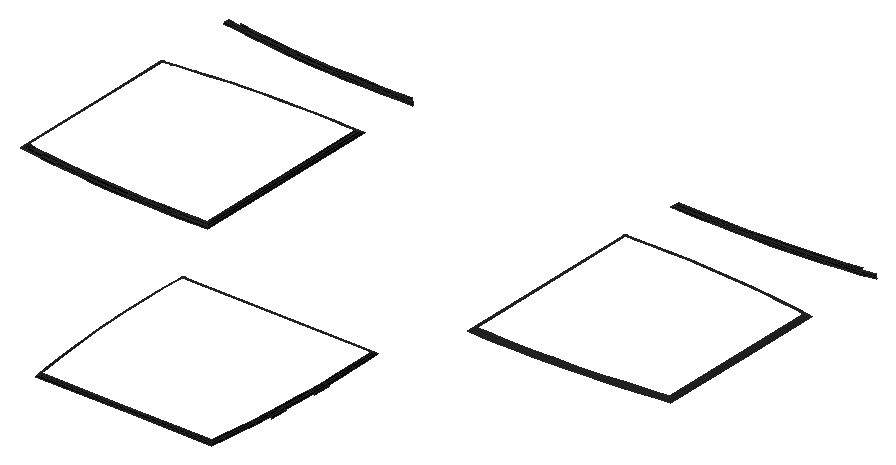
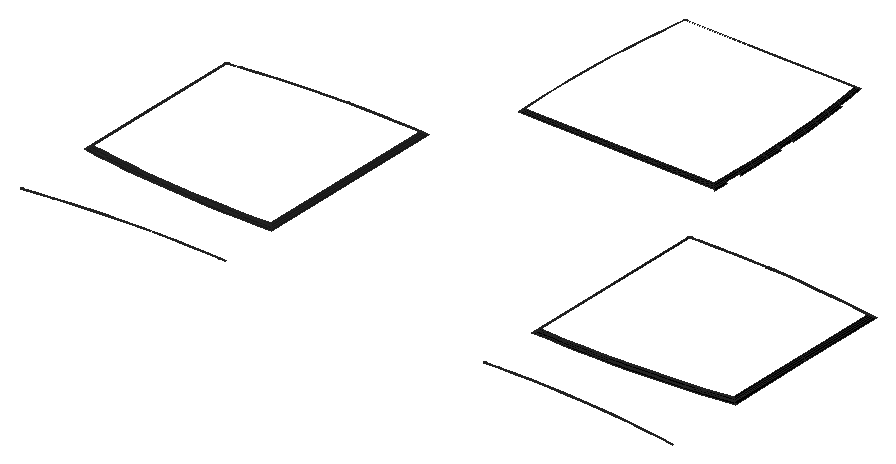
# SketchUp Ruby script. Lengths in inches.
U = 1.inch
M = Sketchup.active_model
def pt(a) = Geom::Point3d.new(a.map { |v| v * U })
def face(e, loops, mat)
  f = e.add_face(loops[0].map { |a| pt(a) })
  loops[1..].each { |l| e.add_face(l.map { |a| pt(a) }).erase! }
  f.material = f.back_material = mat if mat
  f
end
# faces: each face lists its corners as indices into pts; further lists are holes
def faces(e, pts, list, mat = nil) = list.each { |f| face(e, (f[0].is_a?(Array) ? f : [f]).map { |l| l.map { |i| pts[i] } }, mat) }
# xy, xz, yz: faces in a plane at the given z, y or x. An outline is a flat list of corners, or four numbers for a rectangle; further outlines are holes
def ring(l) = l.size == 4 ? [[l[0], l[1]], [l[2], l[1]], [l[2], l[3]], [l[0], l[3]]] : l.each_slice(2).to_a
def flat(e, list, mat, &to3) = list.each { |f| face(e, (f[0].is_a?(Array) ? f : [f]).map { |l| ring(l).map { |u, v| to3.(u, v) } }, mat) }
def xy(e, z, list, mat = nil) = flat(e, list, mat) { |x, y| [x, y, z] }
def xz(e, y, list, mat = nil) = flat(e, list, mat) { |x, z| [x, y, z] }
def yz(e, x, list, mat = nil) = flat(e, list, mat) { |y, z| [x, y, z] }
def lines(e, pts, list) = list.each { |a, b| e.add_line(pt(pts[a]), pt(pts[b])) }
# prism: a flat outline (further loops are holes) pulled along v
def prism(e, loops, v, mat = nil)
  f = face(e, loops, mat); d = Geom::Vector3d.new(v.map { |x| x * U })
  f.pushpull(f.normal.samedirection?(d) ? d.length : -d.length)
end
def box(e, o, s, mat = nil) = prism(e, [[o, [o[0] + s[0], o[1], o[2]], [o[0] + s[0], o[1] + s[1], o[2]], [o[0], o[1] + s[1], o[2]]]], [0, 0, s[2]], mat)
def at(x, y, z, deg = 0) = Geom::Transformation.translation(pt([x, y, z])) * Geom::Transformation.rotation(ORIGIN, Z_AXIS, deg.degrees)
def axes(o, x, y, z) = Geom::Transformation.new([*x, 0, *y, 0, *z, 0, *pt(o).to_a, 1])
def part(name) = M.definitions.add(name)
# library, detail: a bought-in or finely detailed component or shape, given as its bounding box
def library(name, o, s) = part(name).tap { |d| box(d.entities, o, s) }
def detail(e, o, s) = box(e.add_group.entities, o, s)
def put(e, d, t, mat = nil) = e.add_instance(d, t).tap { |i| i.material = mat if mat }
def group(e, t, mat = nil) = e.add_group.tap { |g| g.transformation = t; g.material = mat if mat }.entities
root = M.entities
M.materials.add("[Color M08]").color = [30, 30, 30]
M.materials.add("[Color M09]").color = [0, 0, 0]
p = [[104.863,65.198,29.641],[104.767,65.189,29.531],[104.95,63.496,29.531],[105.047,63.507,29.641],[104.708,66.892,29.641],[104.611,66.884,29.531],
  [104.58,68.589,29.641],[104.484,68.583,29.531],[124.24,68.583,29.531],[124.143,68.589,29.641],[124.016,66.892,29.641],[124.113,66.884,29.531],
  [104.481,70.287,29.641],[104.384,70.283,29.531],[104.313,71.986,29.531],[104.271,73.686,29.531],[104.368,73.688,29.641],[104.41,71.99,29.641],
  [124.453,73.686,29.531],[124.41,71.986,29.531],[124.313,71.99,29.641],[124.356,73.688,29.641],[104.257,75.389,29.531],[104.354,75.389,29.641],
  [104.27,77.092,29.531],[104.368,77.09,29.641],[104.41,78.791,29.641],[104.313,78.794,29.531],[104.374,80.275,29.531],[104.467,80.178,29.641],
  [91.302,113.311,29.531],[93.002,113.24,29.531],[93.004,113.337,29.641],[91.307,113.408,29.641],[94.706,113.197,29.531],[93.006,113.24,29.531],
  [93.01,113.337,29.641],[94.708,113.294,29.641],[96.409,113.28,29.641],[96.409,113.183,29.531],[98.11,113.294,29.641],[98.112,113.197,29.531],
  [99.811,113.336,29.641],[99.814,113.239,29.531],[101.197,113.394,29.641],[101.294,113.3,29.531],[128.913,113.336,29.641],[128.91,113.239,29.531],
  [127.429,113.3,29.531],[127.526,113.394,29.641],[130.614,113.294,29.641],[130.612,113.197,29.531],[132.315,113.28,29.641],[132.315,113.183,29.531],
  [134.016,113.294,29.641],[134.018,113.197,29.531],[135.718,113.24,29.531],[135.714,113.337,29.641],[135.72,113.337,29.641],[135.722,113.24,29.531],
  [137.421,113.311,29.531],[137.417,113.408,29.641],[89.609,113.507,29.641],[89.602,113.41,29.531],[139.121,113.41,29.531],[139.115,113.507,29.641],
  [87.912,113.634,29.641],[87.904,113.537,29.531],[140.82,113.537,29.531],[140.811,113.634,29.641],[86.218,113.79,29.641],[86.208,113.693,29.531],
  [142.515,113.693,29.531],[142.506,113.79,29.641],[84.527,113.973,29.641],[84.515,113.877,29.531],[144.208,113.877,29.531],[144.197,113.973,29.641],
  [82.839,114.185,29.641],[82.826,114.088,29.531],[145.898,114.088,29.531],[145.885,114.185,29.641],[81.435,114.384,29.641],[81.338,114.3,29.531],
  [147.386,114.3,29.531],[147.289,114.384,29.641],[105.368,61.834,29.739],[105.258,61.819,29.641],[105.458,60.415,29.641],[105.554,60.526,29.739],
  [114.362,60.415,29.641],[114.362,60.526,29.739],[123.266,60.415,29.641],[123.17,60.526,29.739],[123.465,61.819,29.641],[123.356,61.834,29.739],
  [105.157,63.52,29.739],[123.677,63.507,29.641],[123.567,63.52,29.739],[104.973,65.209,29.739],[123.86,65.198,29.641],[123.75,65.209,29.739],
  [104.818,66.902,29.739],[123.906,66.902,29.739],[104.691,68.596,29.739],[124.033,68.596,29.739],[104.592,70.293,29.739],[124.242,70.287,29.641],
  [124.132,70.293,29.739],[104.411,71.984,29.641],[104.521,71.987,29.739],[124.313,71.984,29.641],[124.202,71.987,29.739],[104.521,71.994,29.739],
  [104.479,73.69,29.739],[124.203,71.994,29.739],[124.245,73.69,29.739],[104.464,75.389,29.739],[124.259,75.389,29.739],[124.37,75.389,29.641],
  [104.478,77.088,29.739],[124.245,77.088,29.739],[124.356,77.09,29.641],[104.52,78.787,29.739],[124.203,78.787,29.739],[124.314,78.791,29.641],
  [104.573,80.067,29.739],[124.15,80.067,29.739],[124.256,80.178,29.641],[91.307,87.502,29.641],[93.004,87.431,29.641],[93.007,87.542,29.739],
  [91.3125,87.612,29.739],[94.708,87.388,29.641],[93.01,87.431,29.641],[93.014,87.541,29.739],[94.709,87.499,29.739],[96.409,87.485,29.739],
  [96.409,87.374,29.641],[98.108,87.499,29.739],[98.11,87.388,29.641],[99.807,87.541,29.739],[99.811,87.43,29.641],[101.087,87.594,29.739],
  [101.197,87.488,29.641],[128.917,87.541,29.739],[128.913,87.43,29.641],[127.526,87.488,29.641],[127.637,87.594,29.739],[130.615,87.499,29.739],
  [130.614,87.388,29.641],[132.315,87.485,29.739],[132.315,87.374,29.641],[134.014,87.499,29.739],[134.016,87.388,29.641],[135.714,87.431,29.641],
  [135.709,87.541,29.739],[135.717,87.542,29.739],[135.72,87.431,29.641],[137.417,87.502,29.641],[137.411,87.612,29.739],[89.616,87.711,29.739],
  [89.609,87.601,29.641],[101.087,107.171,29.739],[101.197,107.277,29.641],[127.526,107.277,29.641],[127.637,107.171,29.739],[139.115,87.601,29.641],
  [139.108,87.711,29.739],[87.921,87.838,29.739],[87.912,87.728,29.641],[140.811,87.728,29.641],[140.802,87.838,29.739],[86.229,87.994,29.739],
  [86.218,87.884,29.641],[142.506,87.884,29.641],[142.495,87.994,29.739],[84.54,88.177,29.739],[84.527,88.067,29.641],[144.197,88.067,29.641],
  [144.184,88.177,29.739],[82.853,88.388,29.739],[82.839,88.279,29.641],[145.885,88.279,29.641],[145.87,88.388,29.739],[81.545,88.575,29.739],
  [81.435,88.479,29.641],[147.289,88.479,29.641],[147.178,88.575,29.739],[81.545,97.382,29.739],[81.435,97.382,29.641],[147.289,97.382,29.641],
  [147.178,97.382,29.739],[81.545,106.19,29.739],[81.435,106.286,29.641],[147.289,106.286,29.641],[147.178,106.19,29.739],[82.853,106.376,29.739],
  [82.839,106.486,29.641],[145.885,106.486,29.641],[145.87,106.376,29.739],[84.54,106.588,29.739],[84.527,106.697,29.641],[144.197,106.697,29.641],
  [144.184,106.588,29.739],[86.229,106.771,29.739],[86.218,106.881,29.641],[142.506,106.881,29.641],[142.495,106.771,29.739],[87.921,106.926,29.739],
  [87.912,107.036,29.641],[140.811,107.036,29.641],[140.802,106.926,29.739],[89.616,107.053,29.739],[89.609,107.164,29.641],[139.115,107.164,29.641],
  [139.108,107.053,29.739],[91.3125,107.152,29.739],[91.307,107.263,29.641],[137.417,107.263,29.641],[137.411,107.152,29.739],[93.004,107.333,29.641],
  [93.007,107.223,29.739],[93.014,107.223,29.739],[93.01,107.334,29.641],[94.708,107.376,29.641],[94.709,107.265,29.739],[98.108,107.266,29.739],
  [98.11,107.377,29.641],[99.811,107.334,29.641],[99.807,107.224,29.739],[128.913,107.334,29.641],[128.917,107.224,29.739],[130.614,107.377,29.641],
  [130.615,107.266,29.739],[134.016,107.376,29.641],[135.714,107.334,29.641],[135.709,107.223,29.739],[134.014,107.265,29.739],[135.72,107.333,29.641],
  [135.717,107.223,29.739],[96.409,107.39,29.641],[96.409,107.28,29.739],[132.315,107.39,29.641],[132.315,107.28,29.739],[93.007,113.448,29.739],
  [91.3125,113.518,29.739],[93.014,113.447,29.739],[94.709,113.405,29.739],[96.409,113.391,29.739],[98.108,113.405,29.739],[99.807,113.447,29.739],
  [101.087,113.5,29.739],[128.917,113.447,29.739],[127.637,113.5,29.739],[130.615,113.405,29.739],[132.315,113.391,29.739],[134.014,113.405,29.739],
  [135.709,113.447,29.739],[135.717,113.448,29.739],[137.411,113.518,29.739],[89.616,113.617,29.739],[139.108,113.617,29.739],[87.921,113.744,29.739],
  [140.802,113.744,29.739],[86.229,113.9,29.739],[142.495,113.9,29.739],[84.54,114.083,29.739],[144.184,114.083,29.739],[82.853,114.294,29.739],
  [145.87,114.294,29.739],[81.545,114.48,29.739],[147.178,114.48,29.739],[105.489,61.85,29.82],[105.66,60.648,29.82],[114.362,60.648,29.82],
  [123.063,60.648,29.82],[123.234,61.85,29.82],[105.278,63.534,29.82],[123.445,63.534,29.82],[105.095,65.222,29.82],[123.629,65.222,29.82],
  [104.94,66.912,29.82],[123.784,66.912,29.82],[104.813,68.604,29.82],[123.911,68.604,29.82],[104.714,70.299,29.82],[124.01,70.299,29.82],
  [104.644,71.99,29.82],[124.08,71.99,29.82],[104.643,72,29.82],[104.601,73.692,29.82],[124.08,72,29.82],[124.123,73.692,29.82],
  [104.587,75.389,29.82],[124.137,75.389,29.82],[104.601,77.086,29.82],[124.123,77.086,29.82],[104.643,78.783,29.82],[124.081,78.783,29.82],
  [104.691,79.945,29.82],[124.033,79.945,29.82],[93.01,87.664,29.82],[91.319,87.735,29.82],[93.019,87.664,29.82],[94.711,87.622,29.82],
  [96.409,87.607,29.82],[98.106,87.621,29.82],[99.803,87.663,29.82],[100.964,87.711,29.82],[128.921,87.663,29.82],[127.759,87.711,29.82],
  [130.617,87.621,29.82],[132.315,87.607,29.82],[134.012,87.622,29.82],[135.704,87.664,29.82],[135.714,87.664,29.82],[137.405,87.735,29.82],
  [89.624,87.833,29.82],[100.964,107.053,29.82],[127.759,107.053,29.82],[139.099,87.833,29.82],[87.932,87.96,29.82],[140.792,87.96,29.82],
  [86.241,88.116,29.82],[142.482,88.116,29.82],[84.554,88.299,29.82],[144.17,88.299,29.82],[82.869,88.51,29.82],[145.854,88.51,29.82],
  [81.668,88.681,29.82],[147.056,88.681,29.82],[81.668,97.382,29.82],[147.056,97.382,29.82],[81.668,106.084,29.82],[147.056,106.084,29.82],
  [82.869,106.255,29.82],[145.854,106.255,29.82],[84.554,106.466,29.82],[144.17,106.466,29.82],[86.241,106.649,29.82],[142.482,106.649,29.82],
  [87.932,106.804,29.82],[140.792,106.804,29.82],[89.624,106.931,29.82],[139.099,106.931,29.82],[91.319,107.03,29.82],[137.405,107.03,29.82],
  [93.01,107.1,29.82],[135.714,107.1,29.82],[93.019,107.101,29.82],[94.711,107.143,29.82],[96.409,107.157,29.82],[98.106,107.144,29.82],
  [99.803,107.101,29.82],[128.921,107.101,29.82],[130.617,107.144,29.82],[132.315,107.157,29.82],[134.012,107.143,29.82],[135.704,107.101,29.82],
  [93.01,113.57,29.82],[91.319,113.641,29.82],[93.019,113.57,29.82],[94.711,113.527,29.82],[96.409,113.513,29.82],[98.106,113.527,29.82],
  [99.803,113.569,29.82],[100.964,113.617,29.82],[128.921,113.569,29.82],[127.759,113.617,29.82],[130.617,113.527,29.82],[132.315,113.513,29.82],
  [134.012,113.527,29.82],[135.704,113.57,29.82],[135.714,113.57,29.82],[137.405,113.641,29.82],[89.624,113.739,29.82],[139.099,113.739,29.82],
  [87.932,113.866,29.82],[140.792,113.866,29.82],[86.241,114.021,29.82],[142.482,114.021,29.82],[84.554,114.205,29.82],[144.17,114.205,29.82],
  [82.869,114.416,29.82],[145.854,114.416,29.82],[81.668,114.587,29.82],[147.056,114.587,29.82],[105.62,61.867,29.885],[105.775,60.78,29.885],
  [114.362,60.78,29.885],[122.949,60.78,29.885],[123.104,61.867,29.885],[105.409,63.549,29.885],[123.314,63.549,29.885],[105.226,65.235,29.885],
  [123.497,65.235,29.885],[105.071,66.923,29.885],[123.652,66.923,29.885],[104.945,68.613,29.885],[123.779,68.613,29.885],[104.846,70.306,29.885],
  [123.878,70.306,29.885],[104.776,71.994,29.885],[123.948,71.994,29.885],[104.775,72.005,29.885],[104.733,73.694,29.885],[123.948,72.005,29.885],
  [123.991,73.694,29.885],[104.719,75.389,29.885],[124.005,75.389,29.885],[104.733,77.084,29.885],[123.991,77.084,29.885],[104.775,78.779,29.885],
  [123.949,78.779,29.885],[104.817,79.8125,29.885],[123.906,79.8125,29.885],[93.025,87.796,29.885],[94.714,87.754,29.885],[96.409,87.739,29.885],
  [98.104,87.753,29.885],[99.799,87.795,29.885],[130.62,87.753,29.885],[128.925,87.795,29.885],[132.315,87.739,29.885],[134.01,87.754,29.885],
  [135.699,87.796,29.885],[91.325,87.866,29.885],[89.633,87.965,29.885],[93.013,87.796,29.885],[100.832,87.838,29.885],[100.832,106.927,29.885],
  [127.891,87.838,29.885],[127.891,106.927,29.885],[135.71,87.796,29.885],[137.398,87.866,29.885],[139.091,87.965,29.885],[87.942,88.092,29.885],
  [140.781,88.092,29.885],[86.254,88.247,29.885],[142.469,88.247,29.885],[84.569,88.43,29.885],[144.155,88.43,29.885],[82.887,88.641,29.885],
  [145.837,88.641,29.885],[81.8,88.795,29.885],[146.924,88.795,29.885],[81.8,97.382,29.885],[146.924,97.382,29.885],[81.8,105.969,29.885],
  [146.924,105.969,29.885],[82.887,106.124,29.885],[145.837,106.124,29.885],[84.569,106.335,29.885],[144.155,106.335,29.885],[86.254,106.518,29.885],
  [142.469,106.518,29.885],[87.942,106.673,29.885],[140.781,106.673,29.885],[89.633,106.799,29.885],[139.091,106.799,29.885],[91.325,106.898,29.885],
  [137.398,106.898,29.885],[93.013,106.969,29.885],[99.799,106.97,29.885],[128.925,106.97,29.885],[135.71,106.969,29.885],[93.025,106.969,29.885],
  [94.714,107.011,29.885],[96.409,107.025,29.885],[98.104,107.012,29.885],[130.62,107.012,29.885],[132.315,107.025,29.885],[134.01,107.011,29.885],
  [135.699,106.969,29.885],[93.025,113.702,29.885],[94.714,113.659,29.885],[96.409,113.645,29.885],[98.104,113.659,29.885],[99.799,113.701,29.885],
  [130.62,113.659,29.885],[128.925,113.701,29.885],[132.315,113.645,29.885],[134.01,113.659,29.885],[135.699,113.702,29.885],[91.325,113.772,29.885],
  [89.633,113.871,29.885],[93.013,113.702,29.885],[100.832,113.744,29.885],[127.891,113.744,29.885],[135.71,113.702,29.885],[137.398,113.772,29.885],
  [139.091,113.871,29.885],[87.942,113.998,29.885],[140.781,113.998,29.885],[86.254,114.153,29.885],[142.469,114.153,29.885],[84.569,114.336,29.885],
  [144.155,114.336,29.885],[82.887,114.546,29.885],[145.837,114.546,29.885],[94.716,87.893,29.933],[96.409,87.879,29.933],[98.102,87.892,29.933],
  [132.315,87.879,29.933],[130.622,87.892,29.933],[134.008,87.893,29.933],[93.017,87.935,29.933],[91.332,88.006,29.933],[93.031,87.935,29.933],
  [99.794,87.934,29.933],[100.693,87.972,29.933],[100.693,106.793,29.933],[128.93,87.934,29.933],[128.031,87.972,29.933],[128.031,106.793,29.933],
  [135.693,87.935,29.933],[135.707,87.935,29.933],[137.391,88.006,29.933],[89.642,88.104,29.933],[139.081,88.104,29.933],[87.954,88.231,29.933],
  [140.77,88.231,29.933],[86.268,88.386,29.933],[142.455,88.386,29.933],[84.585,88.568,29.933],[144.138,88.568,29.933],[82.905,88.779,29.933],
  [145.818,88.779,29.933],[81.939,88.916,29.933],[146.785,88.916,29.933],[81.939,97.382,29.933],[146.785,97.382,29.933],[81.939,105.848,29.933],
  [146.785,105.848,29.933],[82.905,105.986,29.933],[145.818,105.986,29.933],[84.585,106.196,29.933],[144.138,106.196,29.933],[86.268,106.379,29.933],
  [142.455,106.379,29.933],[87.954,106.534,29.933],[140.77,106.534,29.933],[89.642,106.66,29.933],[139.081,106.66,29.933],[91.332,106.759,29.933],
  [137.391,106.759,29.933],[93.017,106.829,29.933],[93.031,106.83,29.933],[94.716,106.872,29.933],[98.102,106.872,29.933],[99.794,106.83,29.933],
  [128.93,106.83,29.933],[130.622,106.872,29.933],[135.693,106.83,29.933],[134.008,106.872,29.933],[135.707,106.829,29.933],[96.409,106.886,29.933],
  [132.315,106.886,29.933]]
faces(root,p,[[0,1,2,3],[4,5,1,0],[6,7,5,4],[8,9,10,11],[12,13,7,6],[14,15,16,17],[18,19,20,21],[16,15,22,23],
  [23,22,24,25],[26,27,28,29],[30,31,32,33],[34,35,36,37],[32,36,35,31],[34,37,38,39],[39,38,40,41],[41,40,42,43],
  [43,42,44,45],[46,47,48,49],[50,51,47,46],[52,53,51,50],[54,55,53,52],[56,55,54,57],[58,57,56,59],[59,60,61,58],
  [30,33,62,63],[61,60,64,65],[63,62,66,67],[65,64,68,69],[67,66,70,71],[69,68,72,73],[71,70,74,75],[73,72,76,77],
  [75,74,78,79],[77,76,80,81],[79,78,82,83],[81,80,84,85],[86,87,88,89],[89,88,90,91],[92,93,91,90],[94,95,93,92],
  [96,3,87,86],[97,98,95,94],[99,0,3,96],[100,101,98,97],[102,4,0,99],[10,103,101,100],[104,6,4,102],[9,105,103,10],
  [106,12,6,104],[107,108,105,9],[109,12,106,110],[107,111,112,108],[110,113,17,109],[17,16,114,113],[112,115,20,111],[21,20,115,116],
  [114,16,23,117],[21,116,118,119],[117,23,25,120],[119,118,121,122],[120,25,26,123],[122,121,124,125],[123,26,29,126],[125,124,127,128],
  [126,29,128,127],[129,130,131,132],[133,134,135,136],[131,135,134,130],[133,136,137,138],[138,137,139,140],[140,139,141,142],[142,141,143,144],
  [129,132,161,162],[163,164,144,143],[162,161,169,170],[170,169,173,174],[174,173,177,178],[178,177,181,182],[182,181,185,186],[186,185,189,190],
  [193,194,190,189],[197,198,194,193],[201,202,198,197],[205,206,202,201],[209,210,206,205],[213,214,210,209],[217,218,214,213],[221,218,217,222],
  [222,223,224,221],[224,225,226,223],[227,228,229,230],[230,229,164,163],[226,225,241,242],[242,241,228,227],[33,32,245,246],[37,36,247,248],
  [245,247,36,32],[37,248,249,38],[38,249,250,40],[40,250,251,42],[42,251,252,44],[253,46,49,254],[255,50,46,253],[256,52,50,255],
  [257,54,52,256],[57,54,257,258],[259,258,57,58],[58,61,260,259],[33,246,261,62],[260,61,65,262],[62,261,263,66],[262,65,69,264],
  [66,263,265,70],[264,69,73,266],[70,265,267,74],[266,73,77,268],[74,267,269,78],[268,77,81,270],[78,269,271,82],[270,81,85,272],
  [273,86,89,274],[274,89,91,275],[93,276,275,91],[95,277,276,93],[278,96,86,273],[98,279,277,95],[280,99,96,278],[101,281,279,98],
  [282,102,99,280],[103,283,281,101],[284,104,102,282],[105,285,283,103],[286,106,104,284],[108,287,285,105],[110,106,286,288],[108,112,289,287],
  [288,290,113,110],[113,114,291,290],[292,289,112,115],[116,115,292,293],[291,114,117,294],[116,293,295,118],[294,117,120,296],[118,295,297,121],
  [296,120,123,298],[121,297,299,124],[298,123,126,300],[124,299,301,127],[300,126,127,301],[132,131,302,303],[136,135,304,305],[304,302,131,135],
  [136,305,306,137],[137,306,307,139],[139,307,308,141],[141,308,309,143],[132,303,318,161],[319,163,143,309],[161,318,322,169],[169,322,324,173],
  [173,324,326,177],[177,326,328,181],[181,328,330,185],[185,330,332,189],[334,193,189,332],[336,197,193,334],[338,201,197,336],[340,205,201,338],
  [342,209,205,340],[344,213,209,342],[346,217,213,344],[222,217,346,348],[348,350,223,222],[223,226,351,350],[351,226,242,352],[352,242,227,353],
  [353,227,230,354],[354,230,163,319],[246,245,360,361],[248,247,362,363],[362,360,245,247],[248,363,364,249],[249,364,365,250],[250,365,366,251],
  [251,366,367,252],[368,253,254,369],[370,255,253,368],[371,256,255,370],[372,257,256,371],[258,257,372,373],[374,373,258,259],[259,260,375,374],
  [246,361,376,261],[375,260,262,377],[261,376,378,263],[377,262,264,379],[263,378,380,265],[379,264,266,381],[265,380,382,267],[381,266,268,383],
  [267,382,384,269],[383,268,270,385],[269,384,386,271],[385,270,272,387],[388,273,274,389],[389,274,275,390],[276,391,390,275],[277,392,391,276],
  [393,278,273,388],[279,394,392,277],[395,280,278,393],[281,396,394,279],[397,282,280,395],[283,398,396,281],[399,284,282,397],[285,400,398,283],
  [401,286,284,399],[287,402,400,285],[288,286,401,403],[287,289,404,402],[405,403,288,290],[290,291,406,405],[404,407,292,289],[293,292,407,408],
  [406,291,294,409],[293,408,410,295],[409,294,296,411],[295,410,412,297],[411,296,298,413],[297,412,414,299],[413,298,300,415],[299,414,416,301],
  [415,300,301,416],[305,304,417,418],[305,418,419,306],[306,419,420,307],[307,420,421,308],[303,427,428,318],[303,302,429,427],[429,417,304,302],
  [308,421,430,309],[431,319,309,430],[318,428,437,322],[322,437,439,324],[324,439,441,326],[326,441,443,328],[328,443,445,330],[330,445,447,332],
  [449,334,332,447],[451,336,334,449],[453,338,336,451],[455,340,338,453],[457,342,340,455],[459,344,342,457],[461,346,344,459],[348,346,461,463],
  [464,354,319,431],[467,463,348,350],[350,351,468,467],[468,351,352,469],[469,352,353,470],[470,353,354,464],[363,362,475,476],[363,476,477,364],
  [364,477,478,365],[365,478,479,366],[480,370,368,481],[482,371,370,480],[483,372,371,482],[373,372,483,484],[361,485,486,376],[361,360,487,485],
  [487,475,362,360],[366,479,488,367],[481,368,369,489],[484,490,374,373],[374,375,491,490],[491,375,377,492],[376,486,493,378],[492,377,379,494],
  [378,493,495,380],[494,379,381,496],[380,495,497,382],[496,381,383,498],[382,497,499,384],[498,383,385,500],[418,501,502,419],[419,502,503,420],
  [427,429,507,508],[418,417,509,501],[509,507,429,417],[420,503,510,421],[421,510,511,430],[512,431,430,511],[427,508,519,428],[428,519,521,437],
  [437,521,523,439],[439,523,525,441],[441,525,527,443],[443,527,529,445],[445,529,531,447],[533,449,447,531],[535,451,449,533],[537,453,451,535],
  [539,455,453,537],[541,457,455,539],[543,459,457,541],[545,461,459,543],[463,461,545,547],[548,547,463,467],[467,468,549,548],[550,470,464,551],
  [551,464,431,512],[549,468,469,557],[557,469,470,550]],"[Color M09]")
faces(root,p,[[145,146,147,148],[149,150,146,145],[151,152,150,149],[153,154,152,151],[155,154,153,156],[157,156,155,158],[158,159,160,157],[148,147,165,166],
  [160,159,167,168],[168,167,171,172],[172,171,175,176],[176,175,179,180],[180,179,183,184],[184,183,187,188],[188,187,191,192],[195,196,192,191],
  [199,200,196,195],[203,204,200,199],[207,208,204,203],[211,212,208,207],[215,216,212,211],[219,220,216,215],[231,232,166,165],[233,234,232,231],
  [235,236,237,238],[219,239,240,220],[240,237,236,239],[243,244,234,233],[235,238,244,243],[310,145,148,311],[312,149,145,310],[313,151,149,312],
  [314,153,151,313],[156,153,314,315],[316,315,156,157],[157,160,317,316],[311,148,166,320],[317,160,168,321],[321,168,172,323],[323,172,176,325],
  [325,176,180,327],[327,180,184,329],[329,184,188,331],[331,188,192,333],[196,335,333,192],[200,337,335,196],[204,339,337,200],[208,341,339,204],
  [212,343,341,208],[216,345,343,212],[220,347,345,216],[220,240,349,347],[232,355,320,166],[234,356,355,232],[244,357,356,234],[238,358,357,244],
  [238,237,359,358],[359,349,240,237],[422,312,310,423],[424,313,312,422],[425,314,313,424],[315,314,425,426],[423,310,311,432],[432,311,320,433],
  [426,434,316,315],[316,317,435,434],[435,317,321,436],[436,321,323,438],[438,323,325,440],[440,325,327,442],[442,327,329,444],[444,329,331,446],
  [446,331,333,448],[335,450,448,333],[337,452,450,335],[339,454,452,337],[341,456,454,339],[343,458,456,341],[345,460,458,343],[347,462,460,345],
  [355,465,433,320],[347,349,466,462],[356,471,465,355],[357,472,471,356],[358,473,472,357],[358,359,474,473],[466,474,359,349],[504,424,422,505],
  [506,425,424,504],[513,423,432,514],[514,432,433,515],[505,422,423,513],[426,425,506,516],[516,517,434,426],[434,435,518,517],[518,435,436,520],
  [520,436,438,522],[522,438,440,524],[524,440,442,526],[526,442,444,528],[528,444,446,530],[530,446,448,532],[450,534,532,448],[452,536,534,450],
  [454,538,536,452],[456,540,538,454],[458,542,540,456],[460,544,542,458],[462,546,544,460],[465,552,515,433],[471,553,552,465],[473,474,554,555],
  [462,466,556,546],[554,556,466,474],[472,558,553,471],[473,555,558,472]],"[Color M08]")
